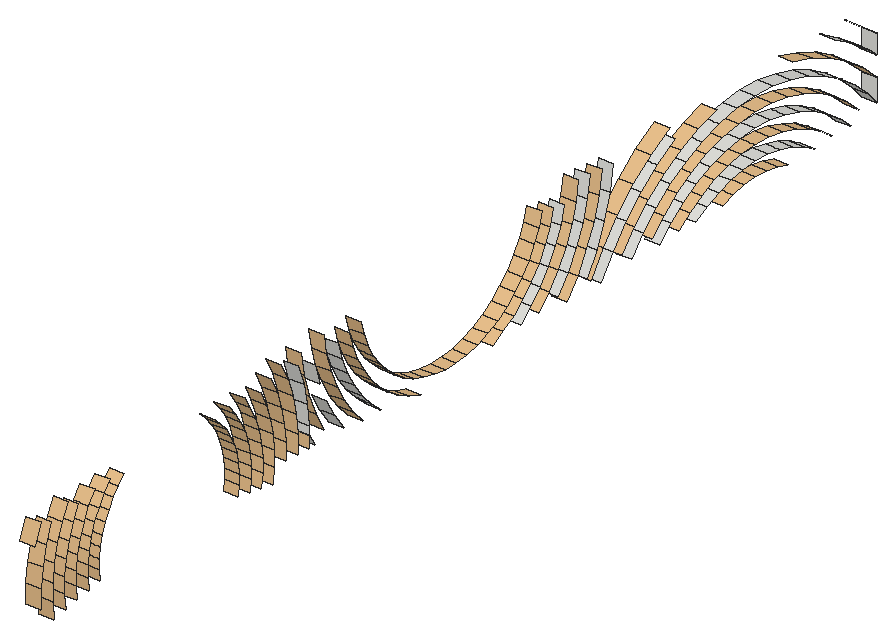
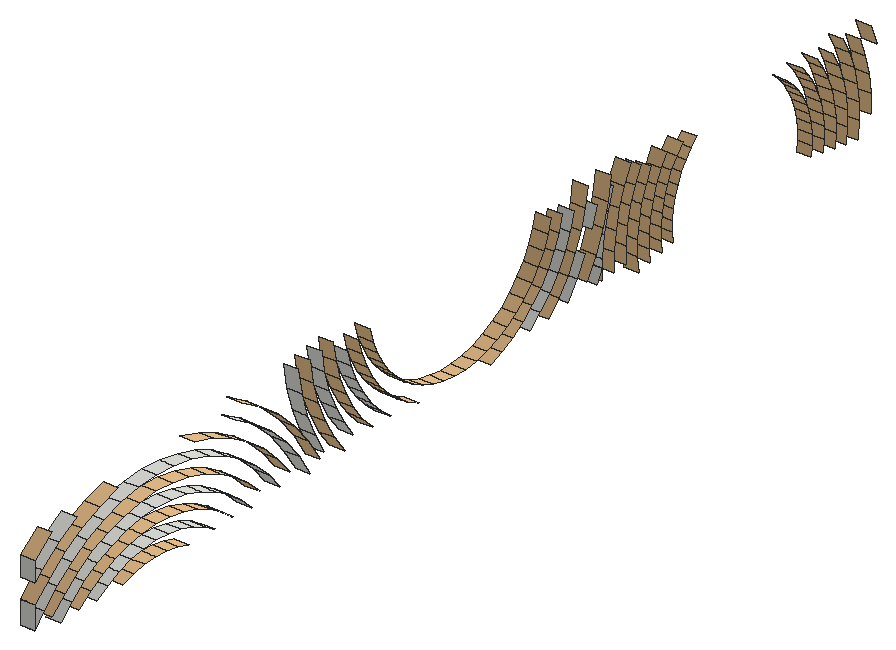
# SketchUp Ruby script. Lengths in inches.
U = 1.inch
M = Sketchup.active_model
def pt(a) = Geom::Point3d.new(a.map { |v| v * U })
def face(e, loops, mat)
  f = e.add_face(loops[0].map { |a| pt(a) })
  loops[1..].each { |l| e.add_face(l.map { |a| pt(a) }).erase! }
  f.material = f.back_material = mat if mat
  f
end
# faces: each face lists its corners as indices into pts; further lists are holes
def faces(e, pts, list, mat = nil) = list.each { |f| face(e, (f[0].is_a?(Array) ? f : [f]).map { |l| l.map { |i| pts[i] } }, mat) }
# xy, xz, yz: faces in a plane at the given z, y or x. An outline is a flat list of corners, or four numbers for a rectangle; further outlines are holes
def ring(l) = l.size == 4 ? [[l[0], l[1]], [l[2], l[1]], [l[2], l[3]], [l[0], l[3]]] : l.each_slice(2).to_a
def flat(e, list, mat, &to3) = list.each { |f| face(e, (f[0].is_a?(Array) ? f : [f]).map { |l| ring(l).map { |u, v| to3.(u, v) } }, mat) }
def xy(e, z, list, mat = nil) = flat(e, list, mat) { |x, y| [x, y, z] }
def xz(e, y, list, mat = nil) = flat(e, list, mat) { |x, z| [x, y, z] }
def yz(e, x, list, mat = nil) = flat(e, list, mat) { |y, z| [x, y, z] }
def lines(e, pts, list) = list.each { |a, b| e.add_line(pt(pts[a]), pt(pts[b])) }
# prism: a flat outline (further loops are holes) pulled along v
def prism(e, loops, v, mat = nil)
  f = face(e, loops, mat); d = Geom::Vector3d.new(v.map { |x| x * U })
  f.pushpull(f.normal.samedirection?(d) ? d.length : -d.length)
end
def box(e, o, s, mat = nil) = prism(e, [[o, [o[0] + s[0], o[1], o[2]], [o[0] + s[0], o[1] + s[1], o[2]], [o[0], o[1] + s[1], o[2]]]], [0, 0, s[2]], mat)
def at(x, y, z, deg = 0) = Geom::Transformation.translation(pt([x, y, z])) * Geom::Transformation.rotation(ORIGIN, Z_AXIS, deg.degrees)
def axes(o, x, y, z) = Geom::Transformation.new([*x, 0, *y, 0, *z, 0, *pt(o).to_a, 1])
def part(name) = M.definitions.add(name)
# library, detail: a bought-in or finely detailed component or shape, given as its bounding box
def library(name, o, s) = part(name).tap { |d| box(d.entities, o, s) }
def detail(e, o, s) = box(e.add_group.entities, o, s)
def put(e, d, t, mat = nil) = e.add_instance(d, t).tap { |i| i.material = mat if mat }
def group(e, t, mat = nil) = e.add_group.tap { |g| g.transformation = t; g.material = mat if mat }.entities
root = M.entities
M.materials.add("images").color = [235, 194, 141]
xy(root,47.6875,[[183.82,117.32,185.82,119.17]],"images")
xz(root,58.04,[[183.82,49.14,185.82,50.54]],"images")
xz(root,82,[[183.82,49.03,185.82,50.42]],"images")
xz(root,191.0625,[[183.82,48.07,185.82,51.16],[183.82,53.9,185.82,56.62]])
p = [[183.82,50.31,46.41],[183.82,50.05,48.72],[185.82,50.05,48.72],[185.82,50.31,46.41],[183.82,113.1,46.42],[183.82,111.14,47.14],
  [185.82,111.14,47.14],[185.82,113.1,46.42],[183.82,87.73,46.57],[183.82,87.98,48.65],[185.82,87.98,48.65],[185.82,87.73,46.57],
  [183.82,52.05,48.83],[183.82,52.28,46.75],[185.82,52.28,46.75],[185.82,52.05,48.83],[183.82,143.99,46.65],[183.82,145.91,49.62],
  [185.82,145.91,49.62],[185.82,143.99,46.65],[183.82,85.99,48.77],[183.82,85.76,46.93],[185.82,85.76,46.93],[185.82,85.99,48.77],
  [183.82,139.92,49.3125],[183.82,138.11,46.89],[185.82,138.11,46.89],[185.82,139.92,49.3125],[183.82,154.02,46.89],[183.82,155.91,48.69],
  [185.82,155.91,48.69],[185.82,154.02,46.89],[183.82,160.21,46.93],[183.82,162.0625,48.02],[185.82,162.0625,48.02],[185.82,160.21,46.93],
  [183.82,166.55,47.5625],[183.82,164.72,47],[185.82,164.72,47],[185.82,166.55,47.5625],[183.82,54.25,47.08],[183.82,54.04,48.93],
  [185.82,54.04,48.93],[185.82,54.25,47.08],[183.82,109.28,48.08],[185.82,109.28,48.08],[183.82,127.21,48.05],[183.82,125.35,47.12],
  [185.82,125.35,47.12],[185.82,127.21,48.05],[183.82,175.96,47.07],[183.82,174.13,47.61],[185.82,174.13,47.61],[185.82,175.96,47.07],
  [183.82,178.61,48.11],[183.82,180.47,47.05],[185.82,180.47,47.05],[185.82,178.61,48.11],[183.82,184.76,48.86],[183.82,186.66,47.08],
  [185.82,186.66,47.08],[185.82,184.76,48.86],[183.82,159.1,48.6],[183.82,157.21,47.17],[185.82,157.21,47.17],[185.82,159.1,48.6],
  [183.82,83.8,47.28],[183.82,83.99,48.9],[185.82,83.99,48.9],[185.82,83.8,47.28],[183.82,149.14,47.25],[183.82,151.1,49.62],
  [185.82,151.1,49.62],[185.82,149.14,47.25],[183.82,183.48,47.32],[183.82,181.5625,48.73],[185.82,181.5625,48.73],[185.82,183.48,47.32],
  [183.82,56.04,49.04],[183.82,56.22,47.42],[185.82,56.22,47.42],[185.82,56.04,49.04],[183.82,82,49.03],[183.82,81.83,47.64],
  [185.82,81.83,47.64],[185.82,82,49.03],[183.82,104.57,49.12],[183.82,106.34,47.62],[185.82,106.34,47.62],[185.82,104.57,49.12],
  [183.82,130.15,47.59],[183.82,131.93,49.07],[185.82,131.93,49.07],[185.82,130.15,47.59],[183.82,135.05,49.47],[183.82,133.3,47.62],
  [185.82,133.3,47.62],[185.82,135.05,49.47],[183.82,144.3,50.81],[183.82,142.25,47.64],[185.82,142.25,47.64],[185.82,144.3,50.81],
  [183.82,168.43,47.9],[185.82,168.43,47.9],[183.82,172.25,47.93],[185.82,172.25,47.93],[183.82,103.19,47.66],[183.82,101.45,49.52],
  [185.82,101.45,49.52],[185.82,103.19,47.66],[183.82,115.48,47.91],[183.82,117.32,47.6875],[185.82,117.32,47.6875],[185.82,115.48,47.91],
  [183.82,119.17,47.6875],[183.82,121.01,47.9],[185.82,121.01,47.9],[185.82,119.17,47.6875],[183.82,58.19,47.76],[183.82,58.04,49.14],
  [185.82,58.04,49.14],[185.82,58.19,47.76],[183.82,113.68,48.34],[185.82,113.68,48.34],[183.82,122.82,48.32],[185.82,122.82,48.32],
  [183.82,170.34,48.03],[185.82,170.34,48.03],[183.82,128.96,49.19],[185.82,128.96,49.19],[183.82,164.03,48.88],[185.82,164.03,48.88],
  [183.82,107.54,49.23],[185.82,107.54,49.23],[183.82,176.64,48.95],[185.82,176.64,48.95],[183.82,189.56,49.84],[183.82,191.0625,48.07],
  [185.82,191.0625,48.07],[185.82,189.56,49.84],[183.82,98.25,50.47],[183.82,99.91,48.24],[185.82,99.91,48.24],[185.82,98.25,50.47],
  [183.82,136.58,48.18],[183.82,138.25,50.41],[185.82,138.25,50.41],[185.82,136.58,48.18],[183.82,141.59,48.21],[183.82,143.21,51.02],
  [185.82,143.21,51.02],[185.82,141.59,48.21],[183.82,93.98,49.89],[183.82,93.97,48.27],[185.82,93.97,48.27],[185.82,93.98,49.89],
  [183.82,94.91,48.28],[185.82,94.91,48.28],[183.82,111.9375,48.97],[185.82,111.9375,48.97],[183.82,124.56,48.95],[185.82,124.56,48.95],
  [183.82,154.62,50.22],[183.82,152.56,48.25],[185.82,152.56,48.25],[185.82,154.62,50.22],[183.82,91.98,48.4],[183.82,91.99,50.95],
  [185.82,91.99,50.95],[185.82,91.98,48.4],[183.82,149.63,50.98],[183.82,147.52,48.4375],[185.82,147.52,48.4375],[185.82,149.63,50.98],
  [183.82,89.99,50.85],[183.82,89.98,48.52],[185.82,89.98,48.52],[185.82,89.99,50.85],[183.82,188.11,48.46],[183.82,186.03,50.4],
  [185.82,186.03,50.4],[185.82,188.11,48.46],[183.82,48.0625,51.17],[183.82,48.05,48.61],[185.82,48.05,48.61],[185.82,48.0625,51.17],
  [183.82,88,50.74],[185.82,88,50.74],[183.82,161.15,49.8],[185.82,161.15,49.8],[183.82,50.06,51.04],[185.82,50.06,51.04],
  [183.82,157.99,50.26],[185.82,157.99,50.26],[183.82,179.5,49.91],[185.82,179.5,49.91],[183.82,52.06,50.92],[185.82,52.06,50.92],
  [183.82,86,50.63],[185.82,86,50.63],[183.82,54.05,50.79],[185.82,54.05,50.79],[183.82,84,50.53],[185.82,84,50.53],
  [183.82,166.08,49.5],[185.82,166.08,49.5],[183.82,182.65,50.41],[185.82,182.65,50.41],[183.82,56.05,50.67],[185.82,56.05,50.67],
  [183.82,110.28,49.81],[185.82,110.28,49.81],[183.82,126.22,49.78],[185.82,126.22,49.78],[183.82,174.58,49.55],[185.82,174.58,49.55],
  [183.82,102.98,50.8],[185.82,102.98,50.8],[183.82,133.52,50.76],[185.82,133.52,50.76],[183.82,105.94,50.57],[185.82,105.94,50.57],
  [183.82,130.56,50.53],[185.82,130.56,50.53],[183.82,141.43,51.92],[185.82,141.43,51.92],[183.82,96.58,49.375],[183.82,95.08,51.99],
  [185.82,95.08,51.99],[185.82,96.58,49.375],[183.82,99.93,51.57],[185.82,99.93,51.57],[183.82,136.58,51.51],[185.82,136.58,51.51],
  [183.82,168.1875,49.89],[185.82,168.1875,49.89],[183.82,148.17,52.35],[185.82,148.17,52.35],[183.82,153.32,51.74],[185.82,153.32,51.74],
  [183.82,172.47,49.91],[185.82,172.47,49.91],[183.82,108.74,50.83],[185.82,108.74,50.83],[183.82,127.77,50.8],[185.82,127.77,50.8],
  [183.82,163.33,50.75],[185.82,163.33,50.75],[183.82,187.31,51.94],[185.82,187.31,51.94],[183.82,93.99,51.06],[185.82,93.99,51.06],
  [183.82,170.33,50.03],[185.82,170.33,50.03],[183.82,177.3125,50.84],[185.82,177.3125,50.84],[183.82,156.89,51.93],[185.82,156.89,51.93],
  [183.82,160.25,51.58],[185.82,160.25,51.58],[183.82,81.85,51.81],[183.82,82,50.42],[185.82,82,50.42],[185.82,81.85,51.81],
  [183.82,139.64,52.82],[185.82,139.64,52.82],[183.82,180.39,51.7],[185.82,180.39,51.7],[183.82,183.74,52.09],[185.82,183.74,52.09],
  [183.82,58.04,50.54],[183.82,58.21,51.93],[185.82,58.21,51.93],[185.82,58.04,50.54],[183.82,83.82,52.15],[185.82,83.82,52.15],
  [183.82,96.87,52.88],[185.82,96.87,52.88],[183.82,131.99,52.05],[185.82,131.99,52.05],[183.82,85.79,52.48],[185.82,85.79,52.48],
  [183.82,104.51,52.09],[185.82,104.51,52.09],[183.82,56.25,52.28],[185.82,56.25,52.28],[183.82,87.76,52.82],[185.82,87.76,52.82],
  [183.82,54.28,52.64],[185.82,54.28,52.64],[183.82,89.73,53.16],[185.82,89.73,53.16],[183.82,101.6,52.67],[185.82,101.6,52.67],
  [183.82,107.32,52.02],[185.82,107.32,52.02],[183.82,129.1875,51.99],[185.82,129.1875,51.99],[183.82,134.91,52.62],[185.82,134.91,52.62],
  [183.82,146.71,53.71],[185.82,146.71,53.71],[183.82,165.6,51.45],[185.82,165.6,51.45],[183.82,175.03,51.5],[185.82,175.03,51.5],
  [183.82,52.31,53],[185.82,52.31,53],[183.82,50.34,53.35],[185.82,50.34,53.35],[183.82,91.71,53.5],[185.82,91.71,53.5],
  [183.82,144.51,54],[185.82,144.51,54],[183.82,152.03,53.27],[185.82,152.03,53.27],[183.82,93.68,53.83],[185.82,93.68,53.83],
  [183.82,48.375,53.71],[185.82,48.375,53.71],[183.82,191,51.23],[183.82,188.58,53.48],[185.82,188.58,53.48],[185.82,191,51.23],
  [183.82,191.0625,51.16],[185.82,191.0625,51.16],[183.82,167.94,51.875],[185.82,167.94,51.875],[183.82,137.86,53.72],[185.82,137.86,53.72],
  [183.82,172.6875,51.9],[185.82,172.6875,51.9],[183.82,98.65,53.78],[185.82,98.65,53.78],[183.82,162.64,52.63],[185.82,162.64,52.63],
  [183.82,155.78,53.59],[185.82,155.78,53.59],[183.82,177.98,52.72],[185.82,177.98,52.72],[183.82,81.53,53.17],[185.82,81.53,53.17],
  [183.82,58.54,53.28],[185.82,58.54,53.28],[183.82,142.63,54.6875],[185.82,142.63,54.6875],[183.82,159.34,53.36],[185.82,159.34,53.36],
  [183.82,170.3125,52.03],[185.82,170.3125,52.03],[183.82,184.83,53.76],[185.82,184.83,53.76],[183.82,93.89,54.76],[185.82,93.89,54.76],
  [183.82,106.05,53.37],[185.82,106.05,53.37],[183.82,130.46,53.33],[185.82,130.46,53.33],[183.82,133.24,53.72],[185.82,133.24,53.72],
  [183.82,83.45,53.73],[185.82,83.45,53.73],[183.82,103.27,53.76],[185.82,103.27,53.76],[183.82,181.27,53.49],[185.82,181.27,53.49],
  [183.82,56.63,53.86],[185.82,56.63,53.86],[183.82,150.73,54.79],[185.82,150.73,54.79],[183.82,85.37,54.3],[185.82,85.37,54.3],
  [183.82,54.72,54.45],[185.82,54.72,54.45],[183.82,136.07,54.62],[185.82,136.07,54.62],[183.82,165.13,53.39],[185.82,165.13,53.39],
  [183.82,100.44,54.67],[185.82,100.44,54.67],[183.82,175.48,53.45],[185.82,175.48,53.45],[183.82,87.29,54.86],[185.82,87.29,54.86],
  [183.82,140.75,55.375],[185.82,140.75,55.375],[183.82,52.8,55.03],[185.82,52.8,55.03],[183.82,81.0625,54.48],[185.82,81.0625,54.48],
  [183.82,89.21,55.42],[185.82,89.21,55.42],[183.82,59.03,54.59],[185.82,59.03,54.59],[183.82,131.57,54.82],[185.82,131.57,54.82],
  [183.82,154.67,55.26],[185.82,154.67,55.26],[183.82,50.89,55.61],[185.82,50.89,55.61],[183.82,104.94,54.86],[185.82,104.94,54.86],
  [183.82,161.94,54.5],[185.82,161.94,54.5],[183.82,167.7,53.86],[185.82,167.7,53.86],[183.82,91.13,55.99],[185.82,91.13,55.99],
  [183.82,172.91,53.89],[185.82,172.91,53.89],[183.82,178.66,54.6],[185.82,178.66,54.6],[183.82,185.92,55.44],[185.82,185.92,55.44],
  [183.82,158.43,55.14],[185.82,158.43,55.14],[183.82,48.98,56.2],[185.82,48.98,56.2],[183.82,82.9,55.26],[185.82,82.9,55.26],
  [183.82,134.29,55.52],[185.82,134.29,55.52],[183.82,138.87,56.0625],[185.82,138.87,56.0625],[183.82,149.4375,56.3125],[185.82,149.4375,56.3125],
  [183.82,93.05,56.55],[185.82,93.05,56.55],[183.82,97.65,56.125],[185.82,97.65,56.125],[183.82,102.23,55.57],[185.82,102.23,55.57],
  [183.82,182.16,55.28],[185.82,182.16,55.28],[183.82,57.19,55.39],[185.82,57.19,55.39],[183.82,170.3,54.03],[185.82,170.3,54.03],
  [183.82,189.86,55.02],[183.82,191.0625,53.9],[185.82,191.0625,53.9],[185.82,189.86,55.02],[183.82,145.44,57.11],[185.82,145.44,57.11],
  [183.82,84.74,56.05],[185.82,84.74,56.05],[183.82,55.36,56.19],[185.82,55.36,56.19],[183.82,80.44,55.73],[185.82,80.44,55.73],
  [183.82,164.66,55.33],[185.82,164.66,55.33],[183.82,59.66,55.83],[185.82,59.66,55.83],[183.82,136.99,56.75],[185.82,136.99,56.75],
  [183.82,175.93,55.4],[185.82,175.93,55.4],[183.82,99.53,56.8],[185.82,99.53,56.8],[183.82,143.5,57.58],[185.82,143.5,57.58],
  [183.82,93.03,57.65],[185.82,93.03,57.65],[183.82,132.5,56.42],[185.82,132.5,56.42],[183.82,153.56,56.92],[185.82,153.56,56.92],
  [183.82,86.58,56.83],[185.82,86.58,56.83],[183.82,104.02,56.46],[185.82,104.02,56.46],[183.82,53.53,56.99],[185.82,53.53,56.99],
  [183.82,187.01,57.12],[185.82,187.01,57.12],[183.82,161.25,56.38],[185.82,161.25,56.38],[183.82,82.18,56.72],[185.82,82.18,56.72],
  [183.82,157.52,56.93],[185.82,157.52,56.93],[183.82,167.45,55.84],[185.82,167.45,55.84],[183.82,179.33,56.49],[185.82,179.33,56.49],
  [183.82,57.93,56.84],[185.82,57.93,56.84],[183.82,88.42,57.61],[185.82,88.42,57.61],[183.82,94.97,58.11],[183.82,95.77,55.44],
  [185.82,95.77,55.44],[185.82,94.97,58.11],[183.82,141.55,58.04],[185.82,141.55,58.04],[183.82,173.13,55.88],[185.82,173.13,55.88],
  [183.82,183.05,57.08],[185.82,183.05,57.08],[183.82,135.11,57.44],[185.82,135.11,57.44],[183.82,51.7,57.8],[185.82,51.7,57.8],
  [183.82,101.41,57.49],[185.82,101.41,57.49],[183.82,79.68,56.9],[185.82,79.68,56.9],[183.82,60.43,57],[185.82,60.43,57],
  [183.82,170.29,56.03],[185.82,170.29,56.03],[183.82,83.92,57.71],[185.82,83.92,57.71],[183.82,90.26,58.4],[185.82,90.26,58.4],
  [183.82,96.92,58.57],[185.82,96.92,58.57],[183.82,139.61,58.5],[185.82,139.61,58.5],[183.82,49.86,58.6],[185.82,49.86,58.6],
  [183.82,56.2,57.85],[185.82,56.2,57.85],[183.82,152.45,58.58],[185.82,152.45,58.58],[183.82,133.24,58.12],[185.82,133.24,58.12],
  [183.82,164.1875,57.28],[185.82,164.1875,57.28],[183.82,103.29,58.17],[185.82,103.29,58.17],[183.82,176.38,57.35],[185.82,176.38,57.35],
  [183.82,92.1,59.18],[185.82,92.1,59.18],[183.82,191.0625,56.62],[183.82,188.1,58.8],[185.82,188.1,58.8],[185.82,191.0625,56.62],
  [183.82,81.29,58.09],[185.82,81.29,58.09],[183.82,137.66,58.97],[185.82,137.66,58.97],[183.82,47.0625,56.78],[183.82,48.03,59.4],
  [185.82,48.03,59.4],[185.82,47.0625,56.78],[183.82,58.83,58.2],[185.82,58.83,58.2],[183.82,85.65,58.71],[185.82,85.65,58.71],
  [183.82,98.87,59.03],[185.82,98.87,59.03],[183.82,78.79,57.97],[185.82,78.79,57.97],[183.82,156.61,58.71],[185.82,156.61,58.71],
  [183.82,160.55,58.25],[185.82,160.55,58.25],[183.82,54.48,58.86],[185.82,54.48,58.86],[183.82,61.33,58.0625],[185.82,61.33,58.0625],
  [183.82,146.01,60.31],[185.82,146.01,60.31],[183.82,180,58.37],[185.82,180,58.37],[183.82,183.93,58.87],[185.82,183.93,58.87],
  [183.82,167.21,57.83],[185.82,167.21,57.83],[183.82,173.35,57.87],[185.82,173.35,57.87],[183.82,135.72,59.43],[185.82,135.72,59.43],
  [183.82,100.8125,59.48],[185.82,100.8125,59.48],[183.82,87.39,59.7],[185.82,87.39,59.7],[183.82,144.02,60.55],[185.82,144.02,60.55],
  [183.82,82.9,59.27],[185.82,82.9,59.27],[183.82,92.51,60.62],[185.82,92.51,60.62],[183.82,52.75,59.87],[185.82,52.75,59.87],
  [183.82,170.28,58.03],[185.82,170.28,58.03],[183.82,57.23,59.4],[185.82,57.23,59.4],[183.82,77.78,58.9375],[185.82,77.78,58.9375],
  [183.82,142.04,60.78],[185.82,142.04,60.78],[183.82,62.35,59.01],[185.82,62.35,59.01],[183.82,80.25,59.34],[185.82,80.25,59.34],
  [183.82,133.77,59.9],[185.82,133.77,59.9],[183.82,59.88,59.44],[185.82,59.88,59.44],[183.82,102.76,59.94],[185.82,102.76,59.94],
  [183.82,163.71,59.22],[185.82,163.71,59.22],[183.82,89.13,60.6875],[185.82,89.13,60.6875],[183.82,176.83,59.3],[185.82,176.83,59.3],
  [183.82,140.05,61.02],[185.82,140.05,61.02],[183.82,96.48,61.08],[185.82,96.48,61.08],[183.82,155.71,60.49],[185.82,155.71,60.49]]
faces(root,p,[[0,1,2,3],[4,5,6,7],[8,9,10,11],[12,13,14,15],[20,21,22,23],[24,25,26,27],[36,37,38,39],[40,41,42,43],
  [5,44,45,6],[46,47,48,49],[50,51,52,53],[62,63,64,65],[66,67,68,69],[74,75,76,77],[78,79,80,81],[82,83,84,85],
  [94,95,96,97],[98,99,100,101],[102,36,39,103],[51,104,105,52],[106,107,108,109],[110,111,112,113],[114,115,116,117],[118,119,120,121],
  [122,110,113,123],[115,124,125,116],[126,102,103,127],[104,126,127,105],[128,46,49,129],[44,132,133,45],[152,153,154,155],[158,122,123,159],
  [124,160,161,125],[162,163,164,165],[166,167,168,169],[170,171,172,173],[174,175,176,177],[178,179,180,181],[182,183,184,185],[9,186,187,10],
  [188,62,65,189],[1,190,191,2],[75,194,195,76],[196,12,15,197],[198,20,23,199],[41,200,201,42],[67,202,203,68],[208,78,81,209],
  [210,158,159,211],[160,212,213,161],[132,220,221,133],[222,128,129,223],[224,24,27,225],[226,227,228,229],[107,230,231,108],[232,94,97,233],
  [242,210,211,243],[212,244,245,213],[246,188,189,247],[194,254,255,195],[256,162,165,257],[260,261,262,263],[179,268,269,180],[270,271,272,273],
  [202,274,275,203],[278,222,223,279],[280,198,199,281],[220,282,283,221],[284,208,209,285],[186,286,287,187],[200,288,289,201],[290,174,177,291],
  [294,242,243,295],[244,296,297,245],[300,98,101,301],[302,246,247,303],[254,304,305,255],[306,196,197,307],[190,308,309,191],[167,310,311,168],
  [314,170,173,315],[318,182,185,319],[320,321,322,323],[324,320,323,325],[326,302,303,327],[328,232,233,329],[304,330,331,305],[230,332,333,231],
  [340,260,263,341],[271,342,343,272],[344,224,225,345],[346,256,257,347],[348,326,327,349],[330,348,349,331],[227,352,353,228],[354,294,295,355],
  [296,356,357,297],[358,278,279,359],[274,360,361,275],[282,362,363,283],[268,364,365,269],[366,284,285,367],[370,280,281,371],[288,372,373,289],
  [286,382,383,287],[386,306,307,387],[388,340,341,389],[390,290,291,391],[342,392,393,343],[356,394,395,357],[396,314,315,397],[308,398,399,309],
  [400,354,355,401],[402,346,347,403],[310,406,407,311],[364,410,411,365],[321,412,413,322],[416,318,319,417],[360,418,419,361],[420,358,359,421],
  [422,328,329,423],[424,300,301,425],[332,428,429,333],[362,430,431,363],[434,366,367,435],[444,370,371,445],[372,446,447,373],[448,388,389,449],
  [450,402,403,451],[392,452,453,393],[410,456,457,411],[460,344,345,461],[352,462,463,353],[394,464,465,395],[382,468,469,383],[470,400,401,471],
  [472,386,387,473],[418,478,479,419],[480,396,397,481],[482,450,451,483],[486,434,435,487],[488,390,391,489],[456,496,497,457],[412,498,499,413],
  [500,420,421,501],[398,502,503,399],[430,504,505,431],[506,448,449,507],[452,508,509,453],[510,482,483,511],[496,510,511,497],[512,444,445,513],
  [406,514,515,407],[428,516,517,429],[518,422,423,519],[520,416,417,521],[446,522,523,447],[524,424,425,525],[464,526,527,465],[530,470,471,531],
  [536,537,538,539],[478,540,541,479],[544,545,546,547],[548,486,487,549],[468,550,551,469],[554,506,507,555],[558,480,481,559],[560,472,473,561],
  [508,562,563,509],[498,566,567,499],[574,500,501,575],[504,576,577,505],[578,488,489,579],[580,460,461,581],[582,512,513,583],[462,584,585,463],
  [502,586,587,503],[522,590,591,523],[592,554,555,593],[562,596,597,563],[540,598,599,541],[526,600,601,527],[602,548,549,603],[604,530,531,605],
  [606,558,559,607],[514,608,609,515],[566,610,611,567],[612,518,519,613],[516,614,615,517],[616,524,525,617]],"images")
faces(root,p,[[16,17,18,19],[28,29,30,31],[32,33,34,35],[54,55,56,57],[58,59,60,61],[70,71,72,73],[86,87,88,89],[90,91,92,93],
  [33,130,131,34],[134,54,57,135],[136,137,138,139],[140,141,142,143],[144,145,146,147],[148,149,150,151],[152,156,157,155],[29,192,193,30],
  [130,204,205,131],[206,58,61,207],[214,134,135,215],[216,86,89,217],[91,218,219,92],[204,234,235,205],[17,236,237,18],[71,238,239,72],
  [240,214,215,241],[248,136,139,249],[250,152,155,251],[234,252,253,235],[252,240,241,253],[192,258,259,193],[145,264,265,146],[266,206,207,267],
  [276,140,143,277],[292,216,217,293],[218,298,299,219],[149,312,313,150],[316,250,251,317],[258,334,335,259],[238,336,337,239],[338,266,267,339],
  [350,248,249,351],[236,368,369,237],[298,374,375,299],[334,376,377,335],[378,292,293,379],[380,338,339,381],[264,384,385,265],[376,404,405,377],
  [408,380,381,409],[336,414,415,337],[426,316,317,427],[432,350,351,433],[404,436,437,405],[436,408,409,437],[438,439,440,441],[312,442,443,313],
  [374,454,455,375],[458,378,379,459],[368,466,467,369],[474,438,441,475],[414,476,477,415],[484,432,433,485],[490,491,492,493],[384,494,495,385],
  [476,528,529,477],[532,484,485,533],[534,426,427,535],[454,542,543,455],[552,458,459,553],[466,556,557,467],[442,564,565,443],[568,474,475,569],
  [528,570,571,529],[572,532,533,573],[570,588,589,571],[588,572,573,589],[494,594,595,495]])
